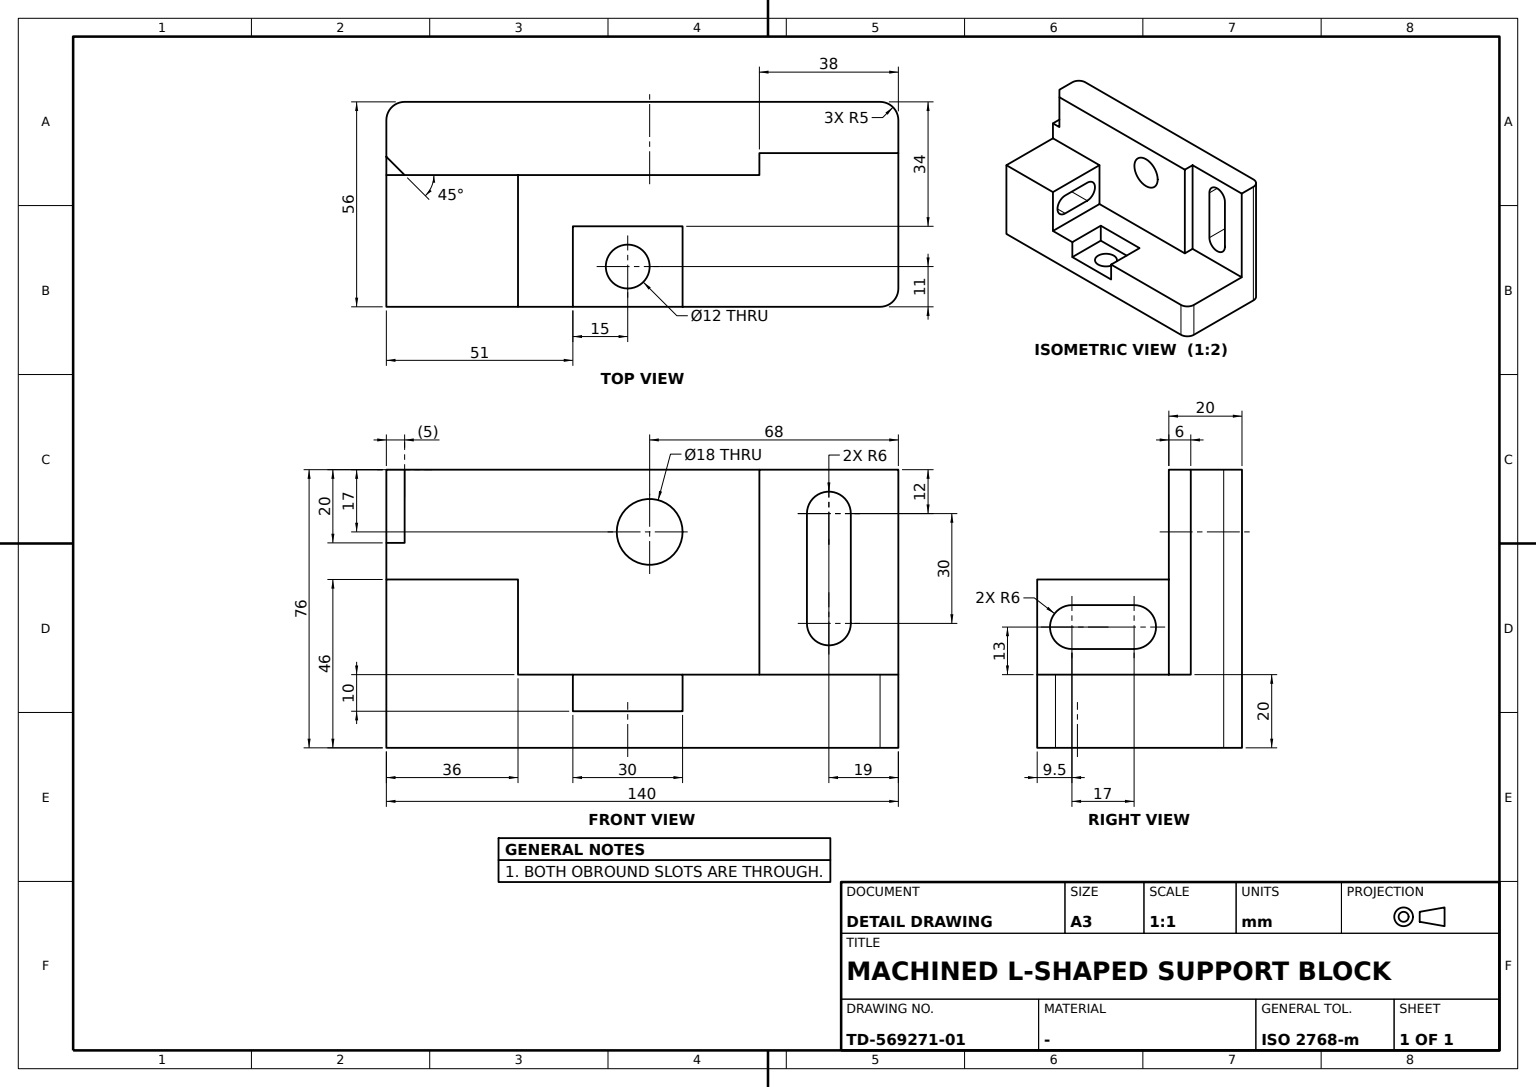
ISO-10303-21;
HEADER;
FILE_DESCRIPTION((''),'2;1');
FILE_NAME('','',(''),(''),'','','');
FILE_SCHEMA(('AUTOMOTIVE_DESIGN'));
ENDSEC;
DATA;
#1=APPLICATION_CONTEXT('');
#2=PRODUCT_CONTEXT('',#1,'mechanical');
#3=PRODUCT('','','',(#2));
#4=PRODUCT_DEFINITION_FORMATION('','',#3);
#5=PRODUCT_DEFINITION_CONTEXT('',#1,'design');
#6=PRODUCT_DEFINITION('','',#4,#5);
#7=PRODUCT_DEFINITION_SHAPE('','',#6);
#8=(LENGTH_UNIT()NAMED_UNIT(*)SI_UNIT(.MILLI.,.METRE.));
#9=(NAMED_UNIT(*)PLANE_ANGLE_UNIT()SI_UNIT($,.RADIAN.));
#10=(NAMED_UNIT(*)SI_UNIT($,.STERADIAN.)SOLID_ANGLE_UNIT());
#11=UNCERTAINTY_MEASURE_WITH_UNIT(LENGTH_MEASURE(1.E-05),#8,'distance_accuracy_value','');
#12=(GEOMETRIC_REPRESENTATION_CONTEXT(3)GLOBAL_UNCERTAINTY_ASSIGNED_CONTEXT((#11))GLOBAL_UNIT_ASSIGNED_CONTEXT((#8,#9,#10))REPRESENTATION_CONTEXT('',''));
#13=CARTESIAN_POINT('',(20.,-65.,76.));
#14=VERTEX_POINT('',#13);
#15=CARTESIAN_POINT('',(15.,-70.,76.));
#16=VERTEX_POINT('',#15);
#17=CARTESIAN_POINT('',(17.5,-67.5,76.));
#18=DIRECTION('',(-0.707106781,-0.707106781,0.));
#19=VECTOR('',#18,1000.);
#20=LINE('',#17,#19);
#21=EDGE_CURVE('',#14,#16,#20,.T.);
#22=ORIENTED_EDGE('',*,*,#21,.F.);
#23=CARTESIAN_POINT('',(20.,32.,76.));
#24=VERTEX_POINT('',#23);
#25=CARTESIAN_POINT('',(20.,-16.5,76.));
#26=DIRECTION('',(0.,1.,0.));
#27=VECTOR('',#26,1000.);
#28=LINE('',#25,#27);
#29=EDGE_CURVE('',#14,#24,#28,.T.);
#30=ORIENTED_EDGE('',*,*,#29,.T.);
#31=CARTESIAN_POINT('',(14.,32.,76.));
#32=VERTEX_POINT('',#31);
#33=CARTESIAN_POINT('',(17.,32.,76.));
#34=DIRECTION('',(-1.,0.,0.));
#35=VECTOR('',#34,1000.);
#36=LINE('',#33,#35);
#37=EDGE_CURVE('',#24,#32,#36,.T.);
#38=ORIENTED_EDGE('',*,*,#37,.T.);
#39=CARTESIAN_POINT('',(14.,70.,76.));
#40=VERTEX_POINT('',#39);
#41=CARTESIAN_POINT('',(14.,51.,76.));
#42=DIRECTION('',(0.,-1.,0.));
#43=VECTOR('',#42,1000.);
#44=LINE('',#41,#43);
#45=EDGE_CURVE('',#40,#32,#44,.T.);
#46=ORIENTED_EDGE('',*,*,#45,.F.);
#47=CARTESIAN_POINT('',(5.,70.,76.));
#48=VERTEX_POINT('',#47);
#49=CARTESIAN_POINT('',(9.5,70.,76.));
#50=DIRECTION('',(1.,0.,0.));
#51=VECTOR('',#50,1000.);
#52=LINE('',#49,#51);
#53=EDGE_CURVE('',#48,#40,#52,.T.);
#54=ORIENTED_EDGE('',*,*,#53,.F.);
#55=CARTESIAN_POINT('',(0.,65.,76.));
#56=VERTEX_POINT('',#55);
#57=CARTESIAN_POINT('',(5.,65.,76.));
#58=DIRECTION('',(0.,0.,-1.));
#59=AXIS2_PLACEMENT_3D('',#57,#58,#50);
#60=CIRCLE('',#59,5.);
#61=EDGE_CURVE('',#56,#48,#60,.T.);
#62=ORIENTED_EDGE('',*,*,#61,.F.);
#63=CARTESIAN_POINT('',(0.,-65.,76.));
#64=VERTEX_POINT('',#63);
#65=CARTESIAN_POINT('',(0.,0.,76.));
#66=LINE('',#65,#27);
#67=EDGE_CURVE('',#64,#56,#66,.T.);
#68=ORIENTED_EDGE('',*,*,#67,.F.);
#69=CARTESIAN_POINT('',(5.,-70.,76.));
#70=VERTEX_POINT('',#69);
#71=CARTESIAN_POINT('',(5.,-65.,76.));
#72=AXIS2_PLACEMENT_3D('',#71,#58,#50);
#73=CIRCLE('',#72,5.);
#74=EDGE_CURVE('',#70,#64,#73,.T.);
#75=ORIENTED_EDGE('',*,*,#74,.F.);
#76=CARTESIAN_POINT('',(10.,-70.,76.));
#77=LINE('',#76,#51);
#78=EDGE_CURVE('',#70,#16,#77,.T.);
#79=ORIENTED_EDGE('',*,*,#78,.T.);
#80=EDGE_LOOP('',(#22,#30,#38,#46,#54,#62,#68,#75,#79));
#81=FACE_OUTER_BOUND('',#80,.T.);
#82=DIRECTION('',(0.,0.,1.));
#83=AXIS2_PLACEMENT_3D('',#65,#82,#50);
#84=PLANE('',#83);
#85=ADVANCED_FACE('',(#81),#84,.T.);
#86=CARTESIAN_POINT('',(51.,-4.,0.));
#87=VERTEX_POINT('',#86);
#88=CARTESIAN_POINT('',(39.,-4.,0.));
#89=VERTEX_POINT('',#88);
#90=CARTESIAN_POINT('',(45.,-4.,0.));
#91=AXIS2_PLACEMENT_3D('',#90,#82,#50);
#92=CIRCLE('',#91,6.);
#93=EDGE_CURVE('',#87,#89,#92,.T.);
#94=ORIENTED_EDGE('',*,*,#93,.F.);
#95=CARTESIAN_POINT('',(51.,-4.,10.));
#96=VERTEX_POINT('',#95);
#97=CARTESIAN_POINT('',(51.,-4.,5.));
#98=VECTOR('',#58,1000.);
#99=LINE('',#97,#98);
#100=EDGE_CURVE('',#96,#87,#99,.T.);
#101=ORIENTED_EDGE('',*,*,#100,.F.);
#102=CARTESIAN_POINT('',(39.,-4.,10.));
#103=VERTEX_POINT('',#102);
#104=CARTESIAN_POINT('',(45.,-4.,10.));
#105=AXIS2_PLACEMENT_3D('',#104,#82,#50);
#106=CIRCLE('',#105,6.);
#107=EDGE_CURVE('',#96,#103,#106,.T.);
#108=ORIENTED_EDGE('',*,*,#107,.T.);
#109=CARTESIAN_POINT('',(39.,-4.,5.));
#110=LINE('',#109,#98);
#111=EDGE_CURVE('',#103,#89,#110,.T.);
#112=ORIENTED_EDGE('',*,*,#111,.T.);
#113=EDGE_LOOP('',(#94,#101,#108,#112));
#114=FACE_OUTER_BOUND('',#113,.T.);
#115=CARTESIAN_POINT('',(45.,-4.,5.));
#116=AXIS2_PLACEMENT_3D('',#115,#58,#50);
#117=CYLINDRICAL_SURFACE('',#116,6.);
#118=ADVANCED_FACE('',(#114),#117,.F.);
#119=CARTESIAN_POINT('',(5.,70.,0.));
#120=VERTEX_POINT('',#119);
#121=CARTESIAN_POINT('',(5.,70.,38.));
#122=VECTOR('',#82,1000.);
#123=LINE('',#121,#122);
#124=EDGE_CURVE('',#120,#48,#123,.T.);
#125=ORIENTED_EDGE('',*,*,#124,.F.);
#126=CARTESIAN_POINT('',(0.,65.,0.));
#127=VERTEX_POINT('',#126);
#128=CARTESIAN_POINT('',(5.,65.,0.));
#129=AXIS2_PLACEMENT_3D('',#128,#82,#50);
#130=CIRCLE('',#129,5.);
#131=EDGE_CURVE('',#120,#127,#130,.T.);
#132=ORIENTED_EDGE('',*,*,#131,.T.);
#133=CARTESIAN_POINT('',(0.,65.,38.));
#134=LINE('',#133,#122);
#135=EDGE_CURVE('',#127,#56,#134,.T.);
#136=ORIENTED_EDGE('',*,*,#135,.T.);
#137=ORIENTED_EDGE('',*,*,#61,.T.);
#138=EDGE_LOOP('',(#125,#132,#136,#137));
#139=FACE_OUTER_BOUND('',#138,.T.);
#140=CARTESIAN_POINT('',(5.,65.,38.));
#141=AXIS2_PLACEMENT_3D('',#140,#58,#34);
#142=CYLINDRICAL_SURFACE('',#141,5.);
#143=ADVANCED_FACE('',(#139),#142,.T.);
#144=CARTESIAN_POINT('',(56.,-70.,46.));
#145=VERTEX_POINT('',#144);
#146=CARTESIAN_POINT('',(56.,-70.,0.));
#147=VERTEX_POINT('',#146);
#148=CARTESIAN_POINT('',(56.,-70.,23.));
#149=LINE('',#148,#98);
#150=EDGE_CURVE('',#145,#147,#149,.T.);
#151=ORIENTED_EDGE('',*,*,#150,.T.);
#152=CARTESIAN_POINT('',(56.,65.,0.));
#153=VERTEX_POINT('',#152);
#154=CARTESIAN_POINT('',(56.,-2.5,0.));
#155=LINE('',#154,#27);
#156=EDGE_CURVE('',#147,#153,#155,.T.);
#157=ORIENTED_EDGE('',*,*,#156,.T.);
#158=CARTESIAN_POINT('',(56.,65.,20.));
#159=VERTEX_POINT('',#158);
#160=CARTESIAN_POINT('',(56.,65.,10.));
#161=LINE('',#160,#98);
#162=EDGE_CURVE('',#159,#153,#161,.T.);
#163=ORIENTED_EDGE('',*,*,#162,.F.);
#164=CARTESIAN_POINT('',(56.,11.,20.));
#165=VERTEX_POINT('',#164);
#166=CARTESIAN_POINT('',(56.,38.,20.));
#167=LINE('',#166,#27);
#168=EDGE_CURVE('',#165,#159,#167,.T.);
#169=ORIENTED_EDGE('',*,*,#168,.F.);
#170=CARTESIAN_POINT('',(56.,11.,10.));
#171=VERTEX_POINT('',#170);
#172=CARTESIAN_POINT('',(56.,11.,15.));
#173=LINE('',#172,#98);
#174=EDGE_CURVE('',#165,#171,#173,.T.);
#175=ORIENTED_EDGE('',*,*,#174,.T.);
#176=CARTESIAN_POINT('',(56.,-19.,10.));
#177=VERTEX_POINT('',#176);
#178=CARTESIAN_POINT('',(56.,-4.,10.));
#179=LINE('',#178,#27);
#180=EDGE_CURVE('',#177,#171,#179,.T.);
#181=ORIENTED_EDGE('',*,*,#180,.F.);
#182=CARTESIAN_POINT('',(56.,-19.,20.));
#183=VERTEX_POINT('',#182);
#184=CARTESIAN_POINT('',(56.,-19.,15.));
#185=LINE('',#184,#98);
#186=EDGE_CURVE('',#183,#177,#185,.T.);
#187=ORIENTED_EDGE('',*,*,#186,.F.);
#188=CARTESIAN_POINT('',(56.,-34.,20.));
#189=VERTEX_POINT('',#188);
#190=CARTESIAN_POINT('',(56.,-26.5,20.));
#191=LINE('',#190,#27);
#192=EDGE_CURVE('',#189,#183,#191,.T.);
#193=ORIENTED_EDGE('',*,*,#192,.F.);
#194=CARTESIAN_POINT('',(56.,-34.,46.));
#195=VERTEX_POINT('',#194);
#196=CARTESIAN_POINT('',(56.,-34.,33.));
#197=LINE('',#196,#122);
#198=EDGE_CURVE('',#189,#195,#197,.T.);
#199=ORIENTED_EDGE('',*,*,#198,.T.);
#200=CARTESIAN_POINT('',(56.,-52.,46.));
#201=LINE('',#200,#27);
#202=EDGE_CURVE('',#145,#195,#201,.T.);
#203=ORIENTED_EDGE('',*,*,#202,.F.);
#204=EDGE_LOOP('',(#151,#157,#163,#169,#175,#181,#187,#193,#199,#203));
#205=FACE_OUTER_BOUND('',#204,.T.);
#206=CARTESIAN_POINT('',(56.,0.,0.));
#207=AXIS2_PLACEMENT_3D('',#206,#34,#82);
#208=PLANE('',#207);
#209=ADVANCED_FACE('',(#205),#208,.F.);
#210=ORIENTED_EDGE('',*,*,#131,.F.);
#211=CARTESIAN_POINT('',(51.,70.,0.));
#212=VERTEX_POINT('',#211);
#213=CARTESIAN_POINT('',(28.,70.,0.));
#214=LINE('',#213,#35);
#215=EDGE_CURVE('',#212,#120,#214,.T.);
#216=ORIENTED_EDGE('',*,*,#215,.F.);
#217=CARTESIAN_POINT('',(51.,65.,0.));
#218=AXIS2_PLACEMENT_3D('',#217,#82,#50);
#219=CIRCLE('',#218,5.);
#220=EDGE_CURVE('',#153,#212,#219,.T.);
#221=ORIENTED_EDGE('',*,*,#220,.F.);
#222=ORIENTED_EDGE('',*,*,#156,.F.);
#223=CARTESIAN_POINT('',(5.,-70.,0.));
#224=VERTEX_POINT('',#223);
#225=CARTESIAN_POINT('',(30.5,-70.,0.));
#226=LINE('',#225,#35);
#227=EDGE_CURVE('',#147,#224,#226,.T.);
#228=ORIENTED_EDGE('',*,*,#227,.T.);
#229=CARTESIAN_POINT('',(0.,-65.,0.));
#230=VERTEX_POINT('',#229);
#231=CARTESIAN_POINT('',(5.,-65.,0.));
#232=AXIS2_PLACEMENT_3D('',#231,#82,#50);
#233=CIRCLE('',#232,5.);
#234=EDGE_CURVE('',#230,#224,#233,.T.);
#235=ORIENTED_EDGE('',*,*,#234,.F.);
#236=CARTESIAN_POINT('',(0.,0.,0.));
#237=LINE('',#236,#27);
#238=EDGE_CURVE('',#230,#127,#237,.T.);
#239=ORIENTED_EDGE('',*,*,#238,.T.);
#240=EDGE_LOOP('',(#210,#216,#221,#222,#228,#235,#239));
#241=FACE_OUTER_BOUND('',#240,.T.);
#242=ORIENTED_EDGE('',*,*,#93,.T.);
#243=EDGE_CURVE('',#89,#87,#92,.T.);
#244=ORIENTED_EDGE('',*,*,#243,.T.);
#245=EDGE_LOOP('',(#242,#244));
#246=FACE_BOUND('',#245,.T.);
#247=AXIS2_PLACEMENT_3D('',#236,#82,#50);
#248=PLANE('',#247);
#249=ADVANCED_FACE('',(#241,#246),#248,.F.);
#250=CARTESIAN_POINT('',(20.,-7.,59.));
#251=VERTEX_POINT('',#250);
#252=CARTESIAN_POINT('',(20.,11.,59.));
#253=VERTEX_POINT('',#252);
#254=CARTESIAN_POINT('',(20.,2.,59.));
#255=AXIS2_PLACEMENT_3D('',#254,#50,#26);
#256=CIRCLE('',#255,9.);
#257=EDGE_CURVE('',#251,#253,#256,.T.);
#258=ORIENTED_EDGE('',*,*,#257,.T.);
#259=CARTESIAN_POINT('',(0.,11.,59.));
#260=VERTEX_POINT('',#259);
#261=CARTESIAN_POINT('',(9.34,11.,59.));
#262=LINE('',#261,#35);
#263=EDGE_CURVE('',#253,#260,#262,.T.);
#264=ORIENTED_EDGE('',*,*,#263,.T.);
#265=CARTESIAN_POINT('',(0.,-7.,59.));
#266=VERTEX_POINT('',#265);
#267=CARTESIAN_POINT('',(0.,2.,59.));
#268=AXIS2_PLACEMENT_3D('',#267,#34,#82);
#269=CIRCLE('',#268,9.);
#270=EDGE_CURVE('',#260,#266,#269,.T.);
#271=ORIENTED_EDGE('',*,*,#270,.T.);
#272=CARTESIAN_POINT('',(9.34,-7.,59.));
#273=LINE('',#272,#35);
#274=EDGE_CURVE('',#251,#266,#273,.T.);
#275=ORIENTED_EDGE('',*,*,#274,.F.);
#276=EDGE_LOOP('',(#258,#264,#271,#275));
#277=FACE_OUTER_BOUND('',#276,.T.);
#278=CARTESIAN_POINT('',(9.34,2.,59.));
#279=AXIS2_PLACEMENT_3D('',#278,#34,#26);
#280=CYLINDRICAL_SURFACE('',#279,9.);
#281=ADVANCED_FACE('',(#277),#280,.F.);
#282=CARTESIAN_POINT('',(29.5,-70.,27.));
#283=VERTEX_POINT('',#282);
#284=CARTESIAN_POINT('',(46.5,-70.,27.));
#285=VERTEX_POINT('',#284);
#286=CARTESIAN_POINT('',(38.,-70.,27.));
#287=LINE('',#286,#51);
#288=EDGE_CURVE('',#283,#285,#287,.T.);
#289=ORIENTED_EDGE('',*,*,#288,.T.);
#290=CARTESIAN_POINT('',(46.5,-34.,27.));
#291=VERTEX_POINT('',#290);
#292=CARTESIAN_POINT('',(46.5,-52.66,27.));
#293=LINE('',#292,#43);
#294=EDGE_CURVE('',#291,#285,#293,.T.);
#295=ORIENTED_EDGE('',*,*,#294,.F.);
#296=CARTESIAN_POINT('',(29.5,-34.,27.));
#297=VERTEX_POINT('',#296);
#298=CARTESIAN_POINT('',(38.,-34.,27.));
#299=LINE('',#298,#35);
#300=EDGE_CURVE('',#291,#297,#299,.T.);
#301=ORIENTED_EDGE('',*,*,#300,.T.);
#302=CARTESIAN_POINT('',(29.5,-52.66,27.));
#303=LINE('',#302,#43);
#304=EDGE_CURVE('',#297,#283,#303,.T.);
#305=ORIENTED_EDGE('',*,*,#304,.T.);
#306=EDGE_LOOP('',(#289,#295,#301,#305));
#307=FACE_OUTER_BOUND('',#306,.T.);
#308=AXIS2_PLACEMENT_3D('',#296,#58,#50);
#309=PLANE('',#308);
#310=ADVANCED_FACE('',(#307),#309,.F.);
#311=CARTESIAN_POINT('',(14.,57.,34.));
#312=VERTEX_POINT('',#311);
#313=CARTESIAN_POINT('',(14.,57.,64.));
#314=VERTEX_POINT('',#313);
#315=CARTESIAN_POINT('',(14.,57.,49.));
#316=LINE('',#315,#122);
#317=EDGE_CURVE('',#312,#314,#316,.T.);
#318=ORIENTED_EDGE('',*,*,#317,.F.);
#319=CARTESIAN_POINT('',(14.,45.,34.));
#320=VERTEX_POINT('',#319);
#321=CARTESIAN_POINT('',(14.,51.,34.));
#322=AXIS2_PLACEMENT_3D('',#321,#50,#26);
#323=CIRCLE('',#322,6.);
#324=EDGE_CURVE('',#320,#312,#323,.T.);
#325=ORIENTED_EDGE('',*,*,#324,.F.);
#326=CARTESIAN_POINT('',(14.,45.,64.));
#327=VERTEX_POINT('',#326);
#328=CARTESIAN_POINT('',(14.,45.,49.));
#329=LINE('',#328,#98);
#330=EDGE_CURVE('',#327,#320,#329,.T.);
#331=ORIENTED_EDGE('',*,*,#330,.F.);
#332=CARTESIAN_POINT('',(14.,51.,64.));
#333=AXIS2_PLACEMENT_3D('',#332,#50,#26);
#334=CIRCLE('',#333,6.);
#335=EDGE_CURVE('',#314,#327,#334,.T.);
#336=ORIENTED_EDGE('',*,*,#335,.F.);
#337=EDGE_LOOP('',(#318,#325,#331,#336));
#338=FACE_BOUND('',#337,.T.);
#339=CARTESIAN_POINT('',(14.,32.,20.));
#340=VERTEX_POINT('',#339);
#341=CARTESIAN_POINT('',(14.,32.,48.));
#342=LINE('',#341,#98);
#343=EDGE_CURVE('',#32,#340,#342,.T.);
#344=ORIENTED_EDGE('',*,*,#343,.T.);
#345=CARTESIAN_POINT('',(14.,70.,20.));
#346=VERTEX_POINT('',#345);
#347=CARTESIAN_POINT('',(14.,51.,20.));
#348=LINE('',#347,#27);
#349=EDGE_CURVE('',#340,#346,#348,.T.);
#350=ORIENTED_EDGE('',*,*,#349,.T.);
#351=CARTESIAN_POINT('',(14.,70.,48.));
#352=LINE('',#351,#122);
#353=EDGE_CURVE('',#346,#40,#352,.T.);
#354=ORIENTED_EDGE('',*,*,#353,.T.);
#355=ORIENTED_EDGE('',*,*,#45,.T.);
#356=EDGE_LOOP('',(#344,#350,#354,#355));
#357=FACE_OUTER_BOUND('',#356,.T.);
#358=CARTESIAN_POINT('',(14.,0.,0.));
#359=AXIS2_PLACEMENT_3D('',#358,#50,#26);
#360=PLANE('',#359);
#361=ADVANCED_FACE('',(#338,#357),#360,.T.);
#362=CARTESIAN_POINT('',(5.,-70.,38.));
#363=LINE('',#362,#122);
#364=EDGE_CURVE('',#224,#70,#363,.T.);
#365=ORIENTED_EDGE('',*,*,#364,.F.);
#366=ORIENTED_EDGE('',*,*,#227,.F.);
#367=ORIENTED_EDGE('',*,*,#150,.F.);
#368=CARTESIAN_POINT('',(20.,-70.,46.));
#369=VERTEX_POINT('',#368);
#370=CARTESIAN_POINT('',(38.,-70.,46.));
#371=LINE('',#370,#51);
#372=EDGE_CURVE('',#369,#145,#371,.T.);
#373=ORIENTED_EDGE('',*,*,#372,.F.);
#374=CARTESIAN_POINT('',(20.,-70.,56.));
#375=VERTEX_POINT('',#374);
#376=CARTESIAN_POINT('',(20.,-70.,51.));
#377=LINE('',#376,#98);
#378=EDGE_CURVE('',#375,#369,#377,.T.);
#379=ORIENTED_EDGE('',*,*,#378,.F.);
#380=CARTESIAN_POINT('',(15.,-70.,56.));
#381=VERTEX_POINT('',#380);
#382=CARTESIAN_POINT('',(17.5,-70.,56.));
#383=LINE('',#382,#35);
#384=EDGE_CURVE('',#375,#381,#383,.T.);
#385=ORIENTED_EDGE('',*,*,#384,.T.);
#386=CARTESIAN_POINT('',(15.,-70.,66.));
#387=LINE('',#386,#98);
#388=EDGE_CURVE('',#16,#381,#387,.T.);
#389=ORIENTED_EDGE('',*,*,#388,.F.);
#390=ORIENTED_EDGE('',*,*,#78,.F.);
#391=EDGE_LOOP('',(#365,#366,#367,#373,#379,#385,#389,#390));
#392=FACE_OUTER_BOUND('',#391,.T.);
#393=CARTESIAN_POINT('',(23.5,-70.,33.));
#394=VERTEX_POINT('',#393);
#395=CARTESIAN_POINT('',(29.5,-70.,39.));
#396=VERTEX_POINT('',#395);
#397=CARTESIAN_POINT('',(29.5,-70.,33.));
#398=AXIS2_PLACEMENT_3D('',#397,#26,#34);
#399=CIRCLE('',#398,6.);
#400=EDGE_CURVE('',#394,#396,#399,.T.);
#401=ORIENTED_EDGE('',*,*,#400,.T.);
#402=CARTESIAN_POINT('',(46.5,-70.,39.));
#403=VERTEX_POINT('',#402);
#404=CARTESIAN_POINT('',(38.,-70.,39.));
#405=LINE('',#404,#35);
#406=EDGE_CURVE('',#403,#396,#405,.T.);
#407=ORIENTED_EDGE('',*,*,#406,.F.);
#408=CARTESIAN_POINT('',(46.5,-70.,33.));
#409=AXIS2_PLACEMENT_3D('',#408,#26,#34);
#410=CIRCLE('',#409,6.);
#411=EDGE_CURVE('',#403,#285,#410,.T.);
#412=ORIENTED_EDGE('',*,*,#411,.T.);
#413=ORIENTED_EDGE('',*,*,#288,.F.);
#414=EDGE_CURVE('',#283,#394,#399,.T.);
#415=ORIENTED_EDGE('',*,*,#414,.T.);
#416=EDGE_LOOP('',(#401,#407,#412,#413,#415));
#417=FACE_BOUND('',#416,.T.);
#418=CARTESIAN_POINT('',(0.,-70.,0.));
#419=AXIS2_PLACEMENT_3D('',#418,#26,#34);
#420=PLANE('',#419);
#421=ADVANCED_FACE('',(#392,#417),#420,.F.);
#422=CARTESIAN_POINT('',(46.5,-34.,39.));
#423=VERTEX_POINT('',#422);
#424=CARTESIAN_POINT('',(46.5,-34.,33.));
#425=AXIS2_PLACEMENT_3D('',#424,#26,#34);
#426=CIRCLE('',#425,6.);
#427=EDGE_CURVE('',#423,#291,#426,.T.);
#428=ORIENTED_EDGE('',*,*,#427,.T.);
#429=ORIENTED_EDGE('',*,*,#294,.T.);
#430=ORIENTED_EDGE('',*,*,#411,.F.);
#431=CARTESIAN_POINT('',(46.5,-52.,39.));
#432=LINE('',#431,#43);
#433=EDGE_CURVE('',#423,#403,#432,.T.);
#434=ORIENTED_EDGE('',*,*,#433,.F.);
#435=EDGE_LOOP('',(#428,#429,#430,#434));
#436=FACE_OUTER_BOUND('',#435,.T.);
#437=CARTESIAN_POINT('',(46.5,-52.66,33.));
#438=AXIS2_PLACEMENT_3D('',#437,#42,#34);
#439=CYLINDRICAL_SURFACE('',#438,6.);
#440=ADVANCED_FACE('',(#436),#439,.F.);
#441=ORIENTED_EDGE('',*,*,#202,.T.);
#442=CARTESIAN_POINT('',(20.,-34.,46.));
#443=VERTEX_POINT('',#442);
#444=CARTESIAN_POINT('',(38.,-34.,46.));
#445=LINE('',#444,#35);
#446=EDGE_CURVE('',#195,#443,#445,.T.);
#447=ORIENTED_EDGE('',*,*,#446,.T.);
#448=CARTESIAN_POINT('',(20.,-52.,46.));
#449=LINE('',#448,#43);
#450=EDGE_CURVE('',#443,#369,#449,.T.);
#451=ORIENTED_EDGE('',*,*,#450,.T.);
#452=ORIENTED_EDGE('',*,*,#372,.T.);
#453=EDGE_LOOP('',(#441,#447,#451,#452));
#454=FACE_OUTER_BOUND('',#453,.T.);
#455=CARTESIAN_POINT('',(0.,0.,46.));
#456=AXIS2_PLACEMENT_3D('',#455,#82,#50);
#457=PLANE('',#456);
#458=ADVANCED_FACE('',(#454),#457,.T.);
#459=ORIENTED_EDGE('',*,*,#263,.F.);
#460=EDGE_CURVE('',#253,#251,#256,.T.);
#461=ORIENTED_EDGE('',*,*,#460,.T.);
#462=ORIENTED_EDGE('',*,*,#274,.T.);
#463=EDGE_CURVE('',#266,#260,#269,.T.);
#464=ORIENTED_EDGE('',*,*,#463,.T.);
#465=EDGE_LOOP('',(#459,#461,#462,#464));
#466=FACE_OUTER_BOUND('',#465,.T.);
#467=ADVANCED_FACE('',(#466),#280,.F.);
#468=CARTESIAN_POINT('',(23.5,-34.,33.));
#469=VERTEX_POINT('',#468);
#470=CARTESIAN_POINT('',(29.5,-34.,33.));
#471=AXIS2_PLACEMENT_3D('',#470,#26,#34);
#472=CIRCLE('',#471,6.);
#473=EDGE_CURVE('',#297,#469,#472,.T.);
#474=ORIENTED_EDGE('',*,*,#473,.T.);
#475=CARTESIAN_POINT('',(23.5,-52.66,33.));
#476=LINE('',#475,#43);
#477=EDGE_CURVE('',#469,#394,#476,.T.);
#478=ORIENTED_EDGE('',*,*,#477,.T.);
#479=ORIENTED_EDGE('',*,*,#414,.F.);
#480=ORIENTED_EDGE('',*,*,#304,.F.);
#481=EDGE_LOOP('',(#474,#478,#479,#480));
#482=FACE_OUTER_BOUND('',#481,.T.);
#483=CARTESIAN_POINT('',(29.5,-52.66,33.));
#484=AXIS2_PLACEMENT_3D('',#483,#42,#34);
#485=CYLINDRICAL_SURFACE('',#484,6.);
#486=ADVANCED_FACE('',(#482),#485,.F.);
#487=CARTESIAN_POINT('',(0.,-65.,38.));
#488=LINE('',#487,#122);
#489=EDGE_CURVE('',#230,#64,#488,.T.);
#490=ORIENTED_EDGE('',*,*,#489,.T.);
#491=ORIENTED_EDGE('',*,*,#67,.T.);
#492=ORIENTED_EDGE('',*,*,#135,.F.);
#493=ORIENTED_EDGE('',*,*,#238,.F.);
#494=EDGE_LOOP('',(#490,#491,#492,#493));
#495=FACE_OUTER_BOUND('',#494,.T.);
#496=ORIENTED_EDGE('',*,*,#270,.F.);
#497=ORIENTED_EDGE('',*,*,#463,.F.);
#498=EDGE_LOOP('',(#496,#497));
#499=FACE_BOUND('',#498,.T.);
#500=CARTESIAN_POINT('',(0.,45.,34.));
#501=VERTEX_POINT('',#500);
#502=CARTESIAN_POINT('',(0.,45.,64.));
#503=VERTEX_POINT('',#502);
#504=CARTESIAN_POINT('',(0.,45.,49.));
#505=LINE('',#504,#122);
#506=EDGE_CURVE('',#501,#503,#505,.T.);
#507=ORIENTED_EDGE('',*,*,#506,.F.);
#508=CARTESIAN_POINT('',(0.,57.,34.));
#509=VERTEX_POINT('',#508);
#510=CARTESIAN_POINT('',(0.,51.,34.));
#511=AXIS2_PLACEMENT_3D('',#510,#34,#82);
#512=CIRCLE('',#511,6.);
#513=EDGE_CURVE('',#509,#501,#512,.T.);
#514=ORIENTED_EDGE('',*,*,#513,.F.);
#515=CARTESIAN_POINT('',(0.,57.,64.));
#516=VERTEX_POINT('',#515);
#517=CARTESIAN_POINT('',(0.,57.,49.));
#518=LINE('',#517,#98);
#519=EDGE_CURVE('',#516,#509,#518,.T.);
#520=ORIENTED_EDGE('',*,*,#519,.F.);
#521=CARTESIAN_POINT('',(0.,51.,64.));
#522=AXIS2_PLACEMENT_3D('',#521,#34,#82);
#523=CIRCLE('',#522,6.);
#524=EDGE_CURVE('',#503,#516,#523,.T.);
#525=ORIENTED_EDGE('',*,*,#524,.F.);
#526=EDGE_LOOP('',(#507,#514,#520,#525));
#527=FACE_BOUND('',#526,.T.);
#528=AXIS2_PLACEMENT_3D('',#236,#34,#82);
#529=PLANE('',#528);
#530=ADVANCED_FACE('',(#495,#499,#527),#529,.T.);
#531=ORIENTED_EDGE('',*,*,#317,.T.);
#532=CARTESIAN_POINT('',(6.34,57.,64.));
#533=LINE('',#532,#35);
#534=EDGE_CURVE('',#314,#516,#533,.T.);
#535=ORIENTED_EDGE('',*,*,#534,.T.);
#536=ORIENTED_EDGE('',*,*,#519,.T.);
#537=CARTESIAN_POINT('',(6.34,57.,34.));
#538=LINE('',#537,#35);
#539=EDGE_CURVE('',#312,#509,#538,.T.);
#540=ORIENTED_EDGE('',*,*,#539,.F.);
#541=EDGE_LOOP('',(#531,#535,#536,#540));
#542=FACE_OUTER_BOUND('',#541,.T.);
#543=AXIS2_PLACEMENT_3D('',#313,#26,#58);
#544=PLANE('',#543);
#545=ADVANCED_FACE('',(#542),#544,.F.);
#546=ORIENTED_EDGE('',*,*,#378,.T.);
#547=ORIENTED_EDGE('',*,*,#450,.F.);
#548=CARTESIAN_POINT('',(20.,-34.,20.));
#549=VERTEX_POINT('',#548);
#550=CARTESIAN_POINT('',(20.,-34.,33.));
#551=LINE('',#550,#122);
#552=EDGE_CURVE('',#549,#443,#551,.T.);
#553=ORIENTED_EDGE('',*,*,#552,.F.);
#554=CARTESIAN_POINT('',(20.,32.,20.));
#555=VERTEX_POINT('',#554);
#556=CARTESIAN_POINT('',(20.,-1.,20.));
#557=LINE('',#556,#27);
#558=EDGE_CURVE('',#549,#555,#557,.T.);
#559=ORIENTED_EDGE('',*,*,#558,.T.);
#560=CARTESIAN_POINT('',(20.,32.,48.));
#561=LINE('',#560,#98);
#562=EDGE_CURVE('',#24,#555,#561,.T.);
#563=ORIENTED_EDGE('',*,*,#562,.F.);
#564=ORIENTED_EDGE('',*,*,#29,.F.);
#565=CARTESIAN_POINT('',(20.,-65.,56.));
#566=VERTEX_POINT('',#565);
#567=CARTESIAN_POINT('',(20.,-65.,66.));
#568=LINE('',#567,#98);
#569=EDGE_CURVE('',#14,#566,#568,.T.);
#570=ORIENTED_EDGE('',*,*,#569,.T.);
#571=CARTESIAN_POINT('',(20.,-67.5,56.));
#572=LINE('',#571,#43);
#573=EDGE_CURVE('',#566,#375,#572,.T.);
#574=ORIENTED_EDGE('',*,*,#573,.T.);
#575=EDGE_LOOP('',(#546,#547,#553,#559,#563,#564,#570,#574));
#576=FACE_OUTER_BOUND('',#575,.T.);
#577=ORIENTED_EDGE('',*,*,#257,.F.);
#578=ORIENTED_EDGE('',*,*,#460,.F.);
#579=EDGE_LOOP('',(#577,#578));
#580=FACE_BOUND('',#579,.T.);
#581=CARTESIAN_POINT('',(20.,0.,76.));
#582=AXIS2_PLACEMENT_3D('',#581,#50,#58);
#583=PLANE('',#582);
#584=ADVANCED_FACE('',(#576,#580),#583,.T.);
#585=CARTESIAN_POINT('',(29.5,-34.,39.));
#586=VERTEX_POINT('',#585);
#587=CARTESIAN_POINT('',(29.5,-52.66,39.));
#588=LINE('',#587,#43);
#589=EDGE_CURVE('',#586,#396,#588,.T.);
#590=ORIENTED_EDGE('',*,*,#589,.F.);
#591=CARTESIAN_POINT('',(38.,-34.,39.));
#592=LINE('',#591,#51);
#593=EDGE_CURVE('',#586,#423,#592,.T.);
#594=ORIENTED_EDGE('',*,*,#593,.T.);
#595=ORIENTED_EDGE('',*,*,#433,.T.);
#596=ORIENTED_EDGE('',*,*,#406,.T.);
#597=EDGE_LOOP('',(#590,#594,#595,#596));
#598=FACE_OUTER_BOUND('',#597,.T.);
#599=AXIS2_PLACEMENT_3D('',#422,#82,#34);
#600=PLANE('',#599);
#601=ADVANCED_FACE('',(#598),#600,.F.);
#602=CARTESIAN_POINT('',(34.,-19.,20.));
#603=VERTEX_POINT('',#602);
#604=CARTESIAN_POINT('',(45.,-19.,20.));
#605=LINE('',#604,#51);
#606=EDGE_CURVE('',#603,#183,#605,.T.);
#607=ORIENTED_EDGE('',*,*,#606,.T.);
#608=ORIENTED_EDGE('',*,*,#186,.T.);
#609=CARTESIAN_POINT('',(34.,-19.,10.));
#610=VERTEX_POINT('',#609);
#611=CARTESIAN_POINT('',(45.,-19.,10.));
#612=LINE('',#611,#51);
#613=EDGE_CURVE('',#610,#177,#612,.T.);
#614=ORIENTED_EDGE('',*,*,#613,.F.);
#615=CARTESIAN_POINT('',(34.,-19.,15.));
#616=LINE('',#615,#98);
#617=EDGE_CURVE('',#603,#610,#616,.T.);
#618=ORIENTED_EDGE('',*,*,#617,.F.);
#619=EDGE_LOOP('',(#607,#608,#614,#618));
#620=FACE_OUTER_BOUND('',#619,.T.);
#621=AXIS2_PLACEMENT_3D('',#182,#42,#34);
#622=PLANE('',#621);
#623=ADVANCED_FACE('',(#620),#622,.F.);
#624=ORIENTED_EDGE('',*,*,#489,.F.);
#625=ORIENTED_EDGE('',*,*,#234,.T.);
#626=ORIENTED_EDGE('',*,*,#364,.T.);
#627=ORIENTED_EDGE('',*,*,#74,.T.);
#628=EDGE_LOOP('',(#624,#625,#626,#627));
#629=FACE_OUTER_BOUND('',#628,.T.);
#630=CARTESIAN_POINT('',(5.,-65.,38.));
#631=AXIS2_PLACEMENT_3D('',#630,#58,#42);
#632=CYLINDRICAL_SURFACE('',#631,5.);
#633=ADVANCED_FACE('',(#629),#632,.T.);
#634=ORIENTED_EDGE('',*,*,#335,.T.);
#635=CARTESIAN_POINT('',(6.34,45.,64.));
#636=LINE('',#635,#35);
#637=EDGE_CURVE('',#327,#503,#636,.T.);
#638=ORIENTED_EDGE('',*,*,#637,.T.);
#639=ORIENTED_EDGE('',*,*,#524,.T.);
#640=ORIENTED_EDGE('',*,*,#534,.F.);
#641=EDGE_LOOP('',(#634,#638,#639,#640));
#642=FACE_OUTER_BOUND('',#641,.T.);
#643=CARTESIAN_POINT('',(6.34,51.,64.));
#644=AXIS2_PLACEMENT_3D('',#643,#34,#26);
#645=CYLINDRICAL_SURFACE('',#644,6.);
#646=ADVANCED_FACE('',(#642),#645,.F.);
#647=ORIENTED_EDGE('',*,*,#573,.F.);
#648=CARTESIAN_POINT('',(17.5,-67.5,56.));
#649=LINE('',#648,#19);
#650=EDGE_CURVE('',#566,#381,#649,.T.);
#651=ORIENTED_EDGE('',*,*,#650,.T.);
#652=ORIENTED_EDGE('',*,*,#384,.F.);
#653=EDGE_LOOP('',(#647,#651,#652));
#654=FACE_OUTER_BOUND('',#653,.T.);
#655=AXIS2_PLACEMENT_3D('',#374,#82,#26);
#656=PLANE('',#655);
#657=ADVANCED_FACE('',(#654),#656,.T.);
#658=ORIENTED_EDGE('',*,*,#192,.T.);
#659=ORIENTED_EDGE('',*,*,#606,.F.);
#660=CARTESIAN_POINT('',(34.,11.,20.));
#661=VERTEX_POINT('',#660);
#662=CARTESIAN_POINT('',(34.,-4.,20.));
#663=LINE('',#662,#43);
#664=EDGE_CURVE('',#661,#603,#663,.T.);
#665=ORIENTED_EDGE('',*,*,#664,.F.);
#666=CARTESIAN_POINT('',(45.,11.,20.));
#667=LINE('',#666,#35);
#668=EDGE_CURVE('',#165,#661,#667,.T.);
#669=ORIENTED_EDGE('',*,*,#668,.F.);
#670=ORIENTED_EDGE('',*,*,#168,.T.);
#671=CARTESIAN_POINT('',(51.,70.,20.));
#672=VERTEX_POINT('',#671);
#673=CARTESIAN_POINT('',(51.,65.,20.));
#674=AXIS2_PLACEMENT_3D('',#673,#58,#34);
#675=CIRCLE('',#674,5.);
#676=EDGE_CURVE('',#672,#159,#675,.T.);
#677=ORIENTED_EDGE('',*,*,#676,.F.);
#678=CARTESIAN_POINT('',(32.5,70.,20.));
#679=LINE('',#678,#51);
#680=EDGE_CURVE('',#346,#672,#679,.T.);
#681=ORIENTED_EDGE('',*,*,#680,.F.);
#682=ORIENTED_EDGE('',*,*,#349,.F.);
#683=CARTESIAN_POINT('',(17.,32.,20.));
#684=LINE('',#683,#35);
#685=EDGE_CURVE('',#555,#340,#684,.T.);
#686=ORIENTED_EDGE('',*,*,#685,.F.);
#687=ORIENTED_EDGE('',*,*,#558,.F.);
#688=CARTESIAN_POINT('',(38.,-34.,20.));
#689=LINE('',#688,#35);
#690=EDGE_CURVE('',#189,#549,#689,.T.);
#691=ORIENTED_EDGE('',*,*,#690,.F.);
#692=EDGE_LOOP('',(#658,#659,#665,#669,#670,#677,#681,#682,#686,#687,#691));
#693=FACE_OUTER_BOUND('',#692,.T.);
#694=CARTESIAN_POINT('',(56.,0.,20.));
#695=AXIS2_PLACEMENT_3D('',#694,#58,#34);
#696=PLANE('',#695);
#697=ADVANCED_FACE('',(#693),#696,.F.);
#698=ORIENTED_EDGE('',*,*,#243,.F.);
#699=ORIENTED_EDGE('',*,*,#111,.F.);
#700=EDGE_CURVE('',#103,#96,#106,.T.);
#701=ORIENTED_EDGE('',*,*,#700,.T.);
#702=ORIENTED_EDGE('',*,*,#100,.T.);
#703=EDGE_LOOP('',(#698,#699,#701,#702));
#704=FACE_OUTER_BOUND('',#703,.T.);
#705=ADVANCED_FACE('',(#704),#117,.F.);
#706=ORIENTED_EDGE('',*,*,#539,.T.);
#707=ORIENTED_EDGE('',*,*,#513,.T.);
#708=CARTESIAN_POINT('',(7.,45.,34.));
#709=LINE('',#708,#35);
#710=EDGE_CURVE('',#320,#501,#709,.T.);
#711=ORIENTED_EDGE('',*,*,#710,.F.);
#712=ORIENTED_EDGE('',*,*,#324,.T.);
#713=EDGE_LOOP('',(#706,#707,#711,#712));
#714=FACE_OUTER_BOUND('',#713,.T.);
#715=CARTESIAN_POINT('',(6.34,51.,34.));
#716=AXIS2_PLACEMENT_3D('',#715,#34,#26);
#717=CYLINDRICAL_SURFACE('',#716,6.);
#718=ADVANCED_FACE('',(#714),#717,.F.);
#719=ORIENTED_EDGE('',*,*,#330,.T.);
#720=ORIENTED_EDGE('',*,*,#710,.T.);
#721=ORIENTED_EDGE('',*,*,#506,.T.);
#722=ORIENTED_EDGE('',*,*,#637,.F.);
#723=EDGE_LOOP('',(#719,#720,#721,#722));
#724=FACE_OUTER_BOUND('',#723,.T.);
#725=AXIS2_PLACEMENT_3D('',#319,#42,#82);
#726=PLANE('',#725);
#727=ADVANCED_FACE('',(#724),#726,.F.);
#728=ORIENTED_EDGE('',*,*,#400,.F.);
#729=ORIENTED_EDGE('',*,*,#477,.F.);
#730=EDGE_CURVE('',#469,#586,#472,.T.);
#731=ORIENTED_EDGE('',*,*,#730,.T.);
#732=ORIENTED_EDGE('',*,*,#589,.T.);
#733=EDGE_LOOP('',(#728,#729,#731,#732));
#734=FACE_OUTER_BOUND('',#733,.T.);
#735=ADVANCED_FACE('',(#734),#485,.F.);
#736=ORIENTED_EDGE('',*,*,#685,.T.);
#737=ORIENTED_EDGE('',*,*,#343,.F.);
#738=ORIENTED_EDGE('',*,*,#37,.F.);
#739=ORIENTED_EDGE('',*,*,#562,.T.);
#740=EDGE_LOOP('',(#736,#737,#738,#739));
#741=FACE_OUTER_BOUND('',#740,.T.);
#742=AXIS2_PLACEMENT_3D('',#554,#42,#82);
#743=PLANE('',#742);
#744=ADVANCED_FACE('',(#741),#743,.F.);
#745=ORIENTED_EDGE('',*,*,#388,.T.);
#746=ORIENTED_EDGE('',*,*,#650,.F.);
#747=ORIENTED_EDGE('',*,*,#569,.F.);
#748=ORIENTED_EDGE('',*,*,#21,.T.);
#749=EDGE_LOOP('',(#745,#746,#747,#748));
#750=FACE_OUTER_BOUND('',#749,.T.);
#751=CARTESIAN_POINT('',(15.,-70.,38.));
#752=DIRECTION('',(0.707106781,-0.707106781,0.));
#753=AXIS2_PLACEMENT_3D('',#751,#752,#58);
#754=PLANE('',#753);
#755=ADVANCED_FACE('',(#750),#754,.T.);
#756=ORIENTED_EDGE('',*,*,#676,.T.);
#757=ORIENTED_EDGE('',*,*,#162,.T.);
#758=ORIENTED_EDGE('',*,*,#220,.T.);
#759=CARTESIAN_POINT('',(51.,70.,10.));
#760=LINE('',#759,#98);
#761=EDGE_CURVE('',#672,#212,#760,.T.);
#762=ORIENTED_EDGE('',*,*,#761,.F.);
#763=EDGE_LOOP('',(#756,#757,#758,#762));
#764=FACE_OUTER_BOUND('',#763,.T.);
#765=CARTESIAN_POINT('',(51.,65.,38.));
#766=AXIS2_PLACEMENT_3D('',#765,#58,#50);
#767=CYLINDRICAL_SURFACE('',#766,5.);
#768=ADVANCED_FACE('',(#764),#767,.T.);
#769=ORIENTED_EDGE('',*,*,#700,.F.);
#770=ORIENTED_EDGE('',*,*,#107,.F.);
#771=EDGE_LOOP('',(#769,#770));
#772=FACE_BOUND('',#771,.T.);
#773=ORIENTED_EDGE('',*,*,#180,.T.);
#774=CARTESIAN_POINT('',(34.,11.,10.));
#775=VERTEX_POINT('',#774);
#776=CARTESIAN_POINT('',(45.,11.,10.));
#777=LINE('',#776,#35);
#778=EDGE_CURVE('',#171,#775,#777,.T.);
#779=ORIENTED_EDGE('',*,*,#778,.T.);
#780=CARTESIAN_POINT('',(34.,-4.,10.));
#781=LINE('',#780,#43);
#782=EDGE_CURVE('',#775,#610,#781,.T.);
#783=ORIENTED_EDGE('',*,*,#782,.T.);
#784=ORIENTED_EDGE('',*,*,#613,.T.);
#785=EDGE_LOOP('',(#773,#779,#783,#784));
#786=FACE_OUTER_BOUND('',#785,.T.);
#787=CARTESIAN_POINT('',(0.,0.,10.));
#788=AXIS2_PLACEMENT_3D('',#787,#82,#50);
#789=PLANE('',#788);
#790=ADVANCED_FACE('',(#772,#786),#789,.T.);
#791=ORIENTED_EDGE('',*,*,#664,.T.);
#792=ORIENTED_EDGE('',*,*,#617,.T.);
#793=ORIENTED_EDGE('',*,*,#782,.F.);
#794=CARTESIAN_POINT('',(34.,11.,15.));
#795=LINE('',#794,#98);
#796=EDGE_CURVE('',#661,#775,#795,.T.);
#797=ORIENTED_EDGE('',*,*,#796,.F.);
#798=EDGE_LOOP('',(#791,#792,#793,#797));
#799=FACE_OUTER_BOUND('',#798,.T.);
#800=AXIS2_PLACEMENT_3D('',#602,#34,#26);
#801=PLANE('',#800);
#802=ADVANCED_FACE('',(#799),#801,.F.);
#803=ORIENTED_EDGE('',*,*,#53,.T.);
#804=ORIENTED_EDGE('',*,*,#353,.F.);
#805=ORIENTED_EDGE('',*,*,#680,.T.);
#806=ORIENTED_EDGE('',*,*,#761,.T.);
#807=ORIENTED_EDGE('',*,*,#215,.T.);
#808=ORIENTED_EDGE('',*,*,#124,.T.);
#809=EDGE_LOOP('',(#803,#804,#805,#806,#807,#808));
#810=FACE_OUTER_BOUND('',#809,.T.);
#811=CARTESIAN_POINT('',(0.,70.,0.));
#812=AXIS2_PLACEMENT_3D('',#811,#26,#34);
#813=PLANE('',#812);
#814=ADVANCED_FACE('',(#810),#813,.T.);
#815=ORIENTED_EDGE('',*,*,#552,.T.);
#816=ORIENTED_EDGE('',*,*,#446,.F.);
#817=ORIENTED_EDGE('',*,*,#198,.F.);
#818=ORIENTED_EDGE('',*,*,#690,.T.);
#819=EDGE_LOOP('',(#815,#816,#817,#818));
#820=FACE_OUTER_BOUND('',#819,.T.);
#821=ORIENTED_EDGE('',*,*,#473,.F.);
#822=ORIENTED_EDGE('',*,*,#300,.F.);
#823=ORIENTED_EDGE('',*,*,#427,.F.);
#824=ORIENTED_EDGE('',*,*,#593,.F.);
#825=ORIENTED_EDGE('',*,*,#730,.F.);
#826=EDGE_LOOP('',(#821,#822,#823,#824,#825));
#827=FACE_BOUND('',#826,.T.);
#828=AXIS2_PLACEMENT_3D('',#548,#42,#50);
#829=PLANE('',#828);
#830=ADVANCED_FACE('',(#820,#827),#829,.F.);
#831=ORIENTED_EDGE('',*,*,#668,.T.);
#832=ORIENTED_EDGE('',*,*,#796,.T.);
#833=ORIENTED_EDGE('',*,*,#778,.F.);
#834=ORIENTED_EDGE('',*,*,#174,.F.);
#835=EDGE_LOOP('',(#831,#832,#833,#834));
#836=FACE_OUTER_BOUND('',#835,.T.);
#837=AXIS2_PLACEMENT_3D('',#660,#26,#50);
#838=PLANE('',#837);
#839=ADVANCED_FACE('',(#836),#838,.F.);
#840=CLOSED_SHELL('',(#85,#118,#143,#209,#249,#281,#310,#361,#421,#440,#458,#467,#486,#530,#545,#584,#601,#623,#633,#646,#657,#697,#705,#718,#727,#735,#744,#755,#768,#790,#802,#814,#830,#839));
#841=MANIFOLD_SOLID_BREP('',#840);
#842=ADVANCED_BREP_SHAPE_REPRESENTATION('',(#841),#12);
#843=SHAPE_DEFINITION_REPRESENTATION(#7,#842);
ENDSEC;
END-ISO-10303-21;
